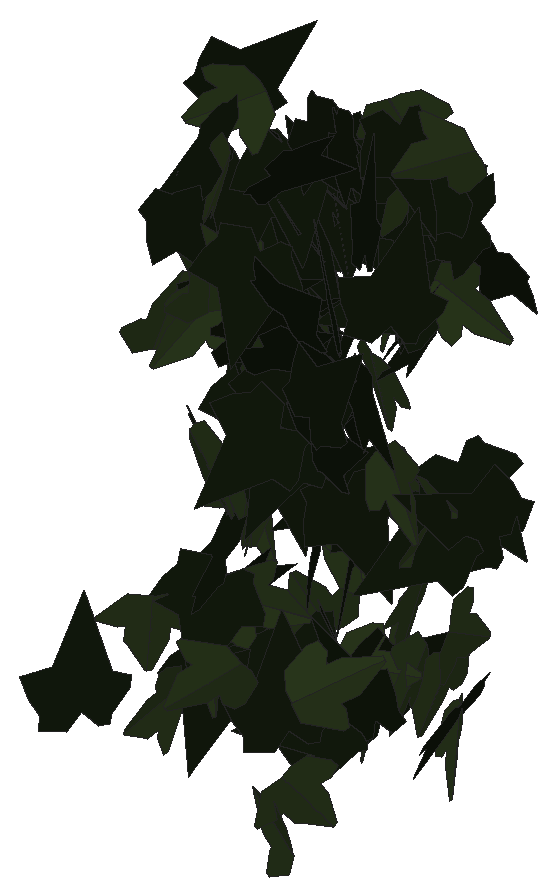
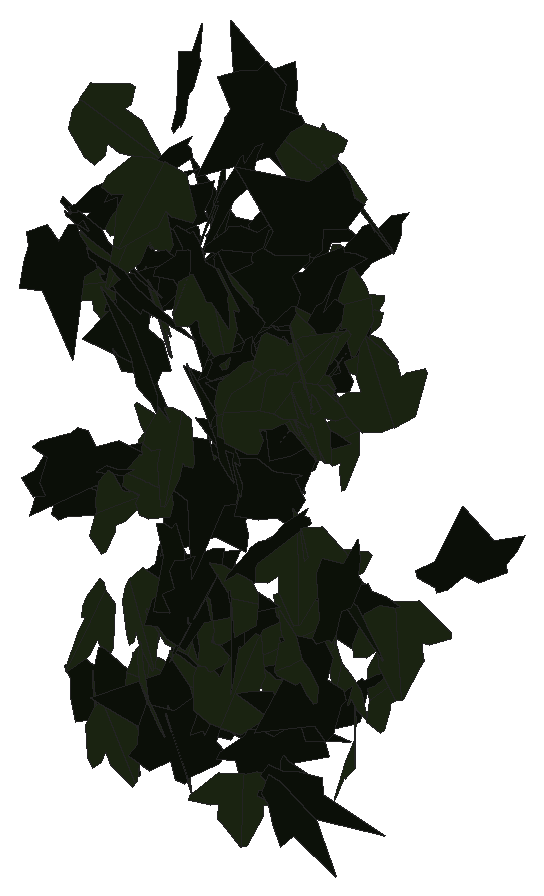
# SketchUp Ruby script. Lengths in inches.
U = 1.inch
M = Sketchup.active_model
def pt(a) = Geom::Point3d.new(a.map { |v| v * U })
def face(e, loops, mat)
  f = e.add_face(loops[0].map { |a| pt(a) })
  loops[1..].each { |l| e.add_face(l.map { |a| pt(a) }).erase! }
  f.material = f.back_material = mat if mat
  f
end
# faces: each face lists its corners as indices into pts; further lists are holes
def faces(e, pts, list, mat = nil) = list.each { |f| face(e, (f[0].is_a?(Array) ? f : [f]).map { |l| l.map { |i| pts[i] } }, mat) }
# xy, xz, yz: faces in a plane at the given z, y or x. An outline is a flat list of corners, or four numbers for a rectangle; further outlines are holes
def ring(l) = l.size == 4 ? [[l[0], l[1]], [l[2], l[1]], [l[2], l[3]], [l[0], l[3]]] : l.each_slice(2).to_a
def flat(e, list, mat, &to3) = list.each { |f| face(e, (f[0].is_a?(Array) ? f : [f]).map { |l| ring(l).map { |u, v| to3.(u, v) } }, mat) }
def xy(e, z, list, mat = nil) = flat(e, list, mat) { |x, y| [x, y, z] }
def xz(e, y, list, mat = nil) = flat(e, list, mat) { |x, z| [x, y, z] }
def yz(e, x, list, mat = nil) = flat(e, list, mat) { |y, z| [x, y, z] }
def lines(e, pts, list) = list.each { |a, b| e.add_line(pt(pts[a]), pt(pts[b])) }
# prism: a flat outline (further loops are holes) pulled along v
def prism(e, loops, v, mat = nil)
  f = face(e, loops, mat); d = Geom::Vector3d.new(v.map { |x| x * U })
  f.pushpull(f.normal.samedirection?(d) ? d.length : -d.length)
end
def box(e, o, s, mat = nil) = prism(e, [[o, [o[0] + s[0], o[1], o[2]], [o[0] + s[0], o[1] + s[1], o[2]], [o[0], o[1] + s[1], o[2]]]], [0, 0, s[2]], mat)
def at(x, y, z, deg = 0) = Geom::Transformation.translation(pt([x, y, z])) * Geom::Transformation.rotation(ORIGIN, Z_AXIS, deg.degrees)
def axes(o, x, y, z) = Geom::Transformation.new([*x, 0, *y, 0, *z, 0, *pt(o).to_a, 1])
def part(name) = M.definitions.add(name)
# library, detail: a bought-in or finely detailed component or shape, given as its bounding box
def library(name, o, s) = part(name).tap { |d| box(d.entities, o, s) }
def detail(e, o, s) = box(e.add_group.entities, o, s)
def put(e, d, t, mat = nil) = e.add_instance(d, t).tap { |i| i.material = mat if mat }
def group(e, t, mat = nil) = e.add_group.tap { |g| g.transformation = t; g.material = mat if mat }.entities
root = M.entities
M.materials.add("efeu1").color = [18, 25, 13]
M.materials.add("efeu2").color = [43, 57, 29]
c1 = part("ivyleaf_9")
p = [[1.54,2.16,1.25],[1.36,2.04,1.19],[-0.21,0.99,0.68],[-0.71,1.11,0.82],[-0.85,0.86,0.67],[-0.8,0.17,0.21],
  [-0.9,-0.01,0.1],[-0.67,-0.16,-0.02],[-0.08,-0.08,-0.05],[-0.03,-0.6,-0.4],[0.65,-0.88,-0.66],[0.83,-0.6,-0.49],
  [1.29,-0.42,-0.43],[1.8125,-0.07,-0.26],[1.21,0.44,0.15]]
faces(c1.entities,p,[[0,1,2,3,4,5,6,7,8,9,10,11,12,13,14]],"efeu1")
c2 = part("ivyleaf_10")
p = [[0,0.5,-0.03],[-0.0625,2.02,-0.43],[-0.19,2.01,-0.46],[-0.54,1.05,-0.29],[-0.52,0.625,-0.18],[-0.83,0.76,-0.28],
  [-1.16,0.64,-0.33],[-1.15,0.33,-0.24],[-0.77,-0.39,0.02],[-0.3,-0.51,0.16],[0.04,-0.48,0.23],[-0.02,2.01,-0.4375],
  [-0.06,2.01,-0.43],[0.04,-0.49,0.23],[0.67,-0.49,0.14],[1.38,0.36,-0.2],[1.375,0.51,-0.24],[0.81,0.65,-0.19],
  [0.62,0.59,-0.15],[0.6,1.09,-0.28],[0.5,1.23,-0.31]]
faces(c2.entities,p,[[0,1,2,3,4,5,6,7,8,9,10],[11,12,0,13,14,15,16,17,18,19,20]],"efeu2")
put(root,c1,axes([35.01,221.78,217.05],[0.13456,-0.26999,0.39875],[0.16922,-0.36111,-0.30161],[0.45084,0.21612,-0.00581]))
put(root,c2,axes([35.25,220.52,219.36],[-0.18393,-0.45885,0.07501],[0.03644,0.06619,0.49426],[-0.46351,0.18729,0.00909]))
put(root,c2,axes([35.36,222.2,220.23],[0.48054,0.03404,-0.13388],[-0.13413,-0.00085,-0.48167],[-0.03302,0.49884,0.00832]))
put(root,c1,axes([35.67,222.1875,214.3125],[-0.42769,-0.02431,0.25786],[-0.25798,-0.00416,-0.42829],[0.02297,-0.49939,-0.00899]))
put(root,c2,axes([35.41,222.34,220.22],[0.05756,0.41296,0.27595],[-0.04863,-0.27177,0.41686],[0.49429,-0.07483,0.00888]))
put(root,c1,axes([35.55,222.26,214.45],[-0.30426,0.30044,-0.25915],[0.17223,-0.1942,-0.42735],[-0.35744,-0.34932,0.01468]))
put(root,c2,axes([35.47,222.05,220.91],[0.25347,-0.43086,0.01047],[0.00775,-0.00759,-0.49988],[0.43092,0.25357,0.00284]))
put(root,c2,axes([35.7,222.04,220.41],[0.21225,0.2584,0.37172],[-0.24741,-0.27761,0.33425],[0.37913,-0.32582,0.01001]))
put(root,c2,axes([35.59,219.91,215.81],[-0.35365,-0.35122,0.03974],[-0.02811,-0.02809,-0.49842],[0.35234,-0.35477,0.00012]))
put(root,c2,axes([35.6875,222.14,220.18],[0.42273,-0.12731,-0.23471],[-0.22624,0.06265,-0.44147],[0.14182,0.47944,-0.00464]))
put(root,c2,axes([35.31,222.22,216.36],[0.27565,-0.05691,0.41325],[0.40121,-0.09944,-0.28132],[0.11421,0.4867,-0.00916]))
put(root,c2,axes([35.55,220.875,214.47],[-0.13494,0.35001,-0.33059],[0.09604,-0.31686,-0.37467],[-0.47177,-0.16462,0.01828]))
put(root,c2,axes([35.78,222.82,220.1],[-0.09609,-0.06927,0.48577],[-0.04461,-0.49171,-0.07894],[0.48865,-0.05852,0.08832]))
put(root,c1,axes([35.47,221.61,222.45],[-0.05533,-0.05972,0.49333],[0.47516,0.13896,0.07012],[-0.14548,0.47657,0.04138]))
put(root,c1,axes([35.78,221.15,215.43],[0.13838,0.29338,0.3805],[0.14932,0.3501,-0.32425],[-0.45668,0.20337,0.00928]))
put(root,c1,axes([35.71,220.23,221.61],[0.15766,-0.33418,-0.33685],[-0.12866,0.31155,-0.3693],[0.45671,0.20313,0.01225]))
put(root,c2,axes([36,220.49,220.04],[0.16571,0.2658,-0.38973],[-0.20211,-0.33324,-0.31321],[-0.42625,0.26134,-0.003]))
put(root,c2,axes([35.93,219.86,214.67],[-0.00988,0.03456,-0.49871],[-0.07298,-0.49356,-0.03275],[-0.49455,0.07215,0.0148]))
put(root,c1,axes([35.77,221.45,219.67],[0.10413,-0.45218,0.18626],[0.03959,-0.18202,-0.46401],[0.48743,0.11138,-0.0021]))
put(root,c1,axes([36.09,217.85,215.47],[-0.32802,-0.23976,0.2914],[0.23696,0.16962,0.4063],[-0.29368,0.40465,0.00235]))
put(root,c1,axes([35.91,221.37,221.5],[-0.11398,-0.48467,-0.04586],[0.01076,0.04458,-0.49789],[0.48672,-0.11449,0.00026]))
put(root,c2,axes([36.29,220.94,222.97],[0.28531,-0.00176,-0.4106],[-0.41049,0.01082,-0.28528],[0.00989,0.49988,0.00473]))
put(root,c2,axes([35.75,220.55,220.79],[-0.25453,0.12719,-0.41114],[0.37694,-0.16461,-0.28428],[-0.20767,-0.45467,-0.01209]))
put(root,c1,axes([36.32,220.41,222.57],[-0.43563,0.24542,-0.00064],[0.00085,0.00021,-0.5],[-0.24542,-0.43563,-0.0006]))
put(root,c1,axes([36.37,220.35,216.59],[-0.34372,0.34921,0.09956],[-0.06978,0.07101,-0.48999],[-0.35635,-0.35073,-0.00008]))
put(root,c2,axes([36.31,222.3125,219.78],[-0.02613,-0.0099,-0.49922],[-0.35119,-0.35499,0.02542],[-0.35494,0.35197,0.0116]))
put(root,c2,axes([36.2,221.17,217.25],[-0.30668,-0.3949,-0.0011],[0.0027,-0.00071,-0.49999],[0.39489,-0.30669,0.00257]))
put(root,c1,axes([36.03,220.64,214.71],[-0.07629,-0.47586,0.13318],[-0.02344,-0.13112,-0.48193],[0.49359,-0.07978,-0.0023]))
put(root,c1,axes([35.74,221.92,221.75],[0.38113,-0.20054,0.25402],[0.22879,-0.11061,-0.4306],[0.2289,0.44447,0.00745]))
put(root,c2,axes([35.93,220.54,215.26],[0.37466,-0.14144,0.29938],[0.28482,-0.09287,-0.40032],[0.16885,0.4705,0.01098]))
put(root,c2,axes([36.16,220.38,220.25],[-0.20375,-0.45,-0.07737],[-0.02016,-0.07578,0.49381],[-0.45616,0.20435,0.01274]))
put(root,c1,axes([35.9,220.68,219.92],[0.16039,0.03716,0.47212],[0.4564,0.1209,-0.16457],[-0.12639,0.48374,0.00487]))
put(root,c1,axes([35.82,221.51,219.67],[0.21229,0.13832,-0.43105],[0.36086,0.23576,0.25337],[0.27333,-0.41867,0.00027]))
put(root,c1,axes([36.23,222.23,220.61],[-0.22899,-0.4393,0.06766],[-0.02428,-0.06364,-0.49534],[0.44382,-0.23014,0.00781]))
put(root,c1,axes([36.57,222.07,221.07],[-0.05323,0.10318,0.48633],[-0.24972,0.41739,-0.11589],[-0.42989,-0.25523,0.0071]))
put(root,c1,axes([36.23,220.45,216.17],[-0.29292,-0.3919,-0.10304],[0.07113,0.07544,-0.48913],[0.39892,-0.30121,0.01156]))
put(root,c1,axes([36.2,221.38,220.15],[-0.1026,-0.40095,-0.28055],[0.09172,0.26582,-0.41344],[0.48069,-0.1363,0.01901]))
put(root,c1,axes([36.1875,221.75,217.62],[0.09283,-0.47949,-0.10711],[-0.01877,0.10546,-0.48839],[0.49095,0.09469,0.00158]))
put(root,c1,axes([36.77,221.64,214.77],[-0.36053,-0.00774,0.34635],[-0.34545,-0.02968,-0.36025],[0.02613,-0.49906,0.01606]))
put(root,c2,axes([36.49,220.81,217.3],[0.28484,-0.36067,-0.19693],[-0.08843,0.1802,-0.45794],[0.40131,0.29571,0.03887]))
put(root,c1,axes([36.22,221.68,221.23],[0.43983,-0.2275,-0.06921],[-0.0612,0.03234,-0.49519],[0.22979,0.44407,0.0006]))
put(root,c2,axes([36.37,222.05,214.07],[0.36359,0.34266,0.01964],[0.01349,0.01432,-0.49961],[-0.34296,0.36384,0.00117]))
put(root,c1,axes([36.33,221.49,214.53],[-0.10411,-0.41087,-0.26523],[0.07854,0.25361,-0.42369],[0.48269,-0.12989,0.01174]))
put(root,c2,axes([36.3,220.73,215.8125],[0.11924,0.12869,0.46821],[0.19159,0.43053,-0.16713],[-0.44618,0.21927,0.05336]))
put(root,c2,axes([36.6,220.03,222.5],[0.29929,-0.38018,-0.12605],[-0.07724,0.09962,-0.48385],[0.39301,0.3091,0.0009]))
put(root,c1,axes([36.51,221.1,218.76],[-0.26653,-0.40408,-0.12522],[0.0652,0.10699,-0.48405],[0.41798,-0.27436,-0.00434]))
put(root,c2,axes([36.33,219.99,218.38],[-0.25445,0.2018,-0.38017],[0.29197,-0.24356,-0.3247],[-0.31624,-0.38724,0.00611]))
put(root,c2,axes([36.81,222.24,221.3],[-0.44574,-0.07255,0.2146],[-0.2119,-0.0339,-0.45161],[0.08008,-0.49355,-0.00052]))
put(root,c2,axes([36.7,221.99,215.09],[-0.27068,-0.3366,-0.25186],[-0.15994,-0.19458,0.43193],[-0.38878,0.31439,-0.00233]))
put(root,c1,axes([36.31,221.84,220.84],[-0.10538,-0.14066,-0.46809],[0.42654,0.20735,-0.15833],[0.23866,-0.43269,0.07629]))
put(root,c1,axes([36.49,221.61,221.96],[-0.17253,-0.4128,-0.22323],[0.10957,0.19583,-0.44682],[0.45632,-0.2031,0.02289]))
put(root,c1,axes([36.91,221.51,216.48],[0.00786,0.0042,-0.49992],[-0.45572,0.20565,-0.00544],[0.20557,0.45573,0.00706]))
put(root,c1,axes([36.48,220.41,219.81],[0.12495,0.38033,-0.29956],[0.06196,0.29427,0.39946],[0.48015,-0.13695,0.02641]))
put(root,c1,axes([36.5,222.03,219.83],[0.10211,-0.35561,0.33632],[0.09972,-0.32124,-0.36995],[0.4792,0.14263,0.00531]))
put(root,c2,axes([36.81,221.11,219.64],[-0.24635,-0.40321,-0.16352],[0.08919,0.13712,-0.47249],[0.42586,-0.26196,0.00436]))
put(root,c1,axes([36.97,222.63,217.01],[-0.08948,-0.05815,-0.48848],[0.02143,-0.49648,0.05518],[-0.49146,-0.01107,0.09135]))
put(root,c2,axes([36.5,222.03,216.75],[0.03504,-0.03536,-0.49752],[0.49358,0.07425,0.02949],[0.0718,-0.49319,0.0401]))
put(root,c2,axes([37.19,219.41,215.69],[-0.22668,-0.21496,0.3904],[-0.29784,-0.25275,-0.31211],[0.33152,-0.37405,-0.01346]))
put(root,c1,axes([36.68,222.48,221.85],[-0.18677,-0.07923,-0.45699],[0.45455,0.06668,-0.19733],[0.09222,-0.48916,0.04712]))
put(root,c1,axes([36.99,221.93,218.52],[0.37446,0.05429,-0.32685],[-0.32677,-0.02106,-0.37786],[-0.0548,0.4966,0.01971]))
put(root,c1,axes([36.7,220.68,217.92],[0.20781,0.43016,-0.14758],[0.06421,0.13288,0.47773],[0.45021,-0.2175,-0.00001]))
put(root,c1,axes([36.87,221.67,218.56],[-0.13441,0.41242,0.24869],[0.05879,-0.24221,0.43345],[0.47799,0.14576,0.01661]))
put(root,c1,axes([36.92,222.125,221.63],[-0.24113,-0.36609,-0.2405],[0.13124,0.20154,-0.43836],[0.41789,-0.27453,-0.0011]))
put(root,c1,axes([36.81,222.54,216.61],[0.24478,-0.19865,-0.3881],[0.2956,-0.25154,0.31519],[-0.32047,-0.38375,-0.0057]))
put(root,c1,axes([36.98,221.34,222.63],[0.23541,-0.24923,-0.36396],[-0.2544,0.26032,-0.3428],[0.36037,0.34658,-0.00424]))
put(root,c1,axes([37.03,221.85,222.25],[0.29545,-0.18178,-0.36009],[-0.30181,0.19651,-0.34683],[0.26762,0.4223,0.0064]))
put(root,c2,axes([37.17,222.16,215.91],[0.46311,0.08908,0.16611],[-0.16527,-0.02,0.47147],[0.09065,-0.49159,0.01092]))
put(root,c1,axes([37.11,220.13,221.33],[-0.35485,-0.31194,-0.16362],[0.12272,0.10821,-0.47247],[0.33018,-0.37548,-0.00024]))
put(root,c1,axes([37.22,220.74,218.51],[-0.45309,-0.16224,-0.13561],[0.12757,0.046,-0.48126],[0.16864,-0.4707,-0.00028]))
put(root,c1,axes([37.25,220.32,218.78],[-0.31351,-0.33549,0.19788],[-0.12223,-0.15645,-0.45889],[0.36983,-0.33611,0.01608]))
put(root,c1,axes([37.02,220.65,219.37],[-0.01592,-0.2587,-0.42758],[0.07691,0.42143,-0.25784],[0.49379,-0.07398,0.02637]))
put(root,c1,axes([37.69,221.2,214.375],[-0.35458,-0.04549,0.34958],[-0.34279,-0.07123,-0.35696],[0.08228,-0.4928,0.01933]))
put(root,c1,axes([37.03,221.84,221.07],[0.10036,-0.07068,-0.4847],[0.47276,-0.11546,0.11473],[-0.12815,-0.48132,0.04366]))
put(root,c1,axes([37.48,221.94,216.79],[-0.00253,0.21702,0.45044],[0.01399,0.4503,-0.21687],[-0.4998,0.01151,-0.00835]))
put(root,c1,axes([37.22,222.03,216.67],[-0.17213,0.07658,-0.46315],[0.414,-0.20779,-0.18822],[-0.22131,-0.44828,0.00813]))
put(root,c1,axes([37.08,220.72,218.34],[-0.11282,-0.00573,0.48707],[0.48582,-0.03758,0.11209],[0.03532,0.49855,0.01405]))
put(root,c2,axes([37.44,222.14,218.97],[-0.4564,0.19198,0.06956],[-0.06539,0.02393,-0.49513],[-0.19344,-0.46105,0.00327]))
put(root,c1,axes([37.09,221.79,214.97],[0.12826,-0.25659,0.40952],[0.16489,-0.37504,-0.28663],[0.45427,0.20858,-0.01159]))
put(root,c1,axes([37.53,220.21,214.67],[-0.44788,-0.12982,0.18042],[0.18076,0.02343,0.46559],[-0.12934,0.48228,0.02594]))
put(root,c1,axes([37.25,220.15,220.05],[0.39119,0.27523,0.14566],[0.11446,0.09043,-0.47825],[-0.2896,0.40752,0.00775]))
put(root,c1,axes([37.56,222.02,214.08],[0.13039,0.09481,0.4733],[-0.40991,-0.23714,0.16043],[0.25489,-0.42986,0.01589]))
put(root,c2,axes([37.55,222,214.46],[0.30567,-0.37979,0.11102],[0.07392,-0.083,-0.48749],[0.38872,0.31443,0.00541]))
put(root,c1,axes([37.51,219.96,222.71],[0.25003,0.33159,0.27844],[0.15182,0.23398,-0.41498],[-0.4055,0.29206,0.01632]))
put(root,c2,axes([37.65,222.3,222.66],[-0.39526,-0.23135,-0.20062],[0.17627,0.09597,-0.45795],[0.2504,-0.43274,0.0057]))
put(root,c2,axes([37.55,222.59,215.34],[0.30843,-0.21713,0.32821],[0.25524,-0.20703,-0.37682],[0.29954,0.39999,-0.01686]))
put(root,c1,axes([37.58,221.67,214.64],[0.09308,0.07847,0.48495],[0.39227,0.28526,-0.12145],[-0.29573,0.40308,-0.00846]))
put(root,c1,axes([37.6,221.3,217.53],[-0.16981,-0.20881,-0.42138],[0.31331,0.28388,-0.26693],[0.35072,-0.3547,0.03443]))
put(root,c2,axes([37.49,221.65,214.9],[0.06926,-0.08453,-0.48791],[0.48165,-0.10287,0.0862],[-0.11496,-0.48195,0.06718]))
put(root,c1,axes([38.36,222.31,220.99],[-0.37146,0.1981,0.26977],[-0.24909,0.10556,-0.42049],[-0.22355,-0.44678,0.02027]))
put(root,c1,axes([37.91,222.13,219.71],[-0.1768,0.43791,0.16425],[0.01378,-0.17064,0.46978],[0.46749,0.17064,0.04827]))
put(root,c2,axes([38.36,219.05,213.79],[-0.0713,0.05399,-0.49194],[-0.35659,0.33903,0.08889],[0.34316,0.36351,-0.00984]))
put(root,c2,axes([38.14,222.59,214.6875],[-0.0622,-0.47456,0.14464],[-0.00553,-0.1451,-0.47845],[0.49608,-0.06112,0.0128]))
put(root,c1,axes([37.97,221.87,221.27],[-0.32515,-0.10967,-0.36367],[0.34397,0.11808,-0.34314],[0.16114,-0.47332,-0.00134]))
put(root,c2,axes([38.09,221.75,220.64],[0.34729,-0.3558,0.05283],[0.03639,-0.0383,-0.4972],[0.35786,0.34919,-0.00071]))
put(root,c1,axes([37.77,220.44,218.71],[0.06331,-0.07543,0.49021],[0.32311,-0.36865,-0.09845],[0.37628,0.32925,0.00207]))
put(root,c1,axes([37.94,221.97,222.63],[0.10056,-0.45864,-0.17187],[-0.01842,0.17179,-0.4692],[0.48944,0.1007,0.01765]))
put(root,c2,axes([38.11,221.99,221.85],[-0.10019,-0.38845,-0.29844],[0.11377,0.27783,-0.39983],[0.47646,-0.14802,0.03272]))
put(root,c1,axes([38.43,221.85,220.49],[-0.33172,-0.14869,0.3433],[-0.29739,-0.17357,-0.36254],[0.22698,-0.44471,0.02672]))
put(root,c1,axes([38.24,221.74,220],[-0.21384,0.36613,-0.265],[-0.13294,0.22924,0.424],[0.43197,0.25179,-0.00069]))
put(root,c1,axes([38.4375,222,220.02],[-0.36926,0.33285,-0.05347],[0.03999,-0.03549,-0.49713],[-0.33474,-0.37142,-0.00041]))
put(root,c2,axes([38.25,221.9,216.12],[0.11579,-0.48512,0.03543],[0.00676,-0.03481,-0.49874],[0.48636,0.11598,-0.00151]))
put(root,c1,axes([38.41,220.08,220.68],[0.02985,-0.23167,0.44208],[-0.0791,0.43508,0.23334],[-0.4928,-0.08387,-0.01068]))
put(root,c2,axes([38.17,221.99,215.03],[0.05261,-0.26268,0.42218],[0.21518,-0.37069,-0.25746],[0.44825,0.20878,0.07404]))
put(root,c1,axes([38.6,222.31,221.88],[-0.19495,-0.41079,-0.20796],[-0.09415,-0.1855,0.45467],[-0.4507,0.21643,-0.00503]))
put(root,c2,axes([38.39,219.21,214.56],[-0.21739,-0.34159,-0.29335],[0.1739,0.23678,-0.40459],[0.41533,-0.27794,0.01586]))
put(root,c2,axes([38.11,221.63,217.71],[-0.01185,-0.03736,0.49846],[0.49204,0.08695,0.01822],[-0.08805,0.49096,0.0347]))
put(root,c2,axes([38.23,221.35,218.13],[0.35751,-0.05917,0.34451],[0.3461,-0.00915,-0.36074],[0.04899,0.4964,0.03441]))
put(root,c1,axes([38.8125,220.31,215.22],[0.11917,-0.11323,0.4722],[-0.35951,0.30627,0.16417],[-0.32642,-0.37865,-0.00841]))
put(root,c1,axes([38.97,222.2,221.5625],[-0.43944,0.1812,0.15512],[-0.14439,0.05675,-0.47532],[-0.18986,-0.46254,0.00245]))
put(root,c2,axes([38.75,221.93,217.29],[0.01137,0.11449,-0.48658],[-0.10023,-0.4763,-0.11442],[-0.48972,0.10014,0.01212]))
put(root,c2,axes([39.14,221.65,222.84],[-0.1938,-0.11519,0.44629],[-0.38489,-0.2259,-0.22545],[0.25357,-0.43093,-0.00112]))
put(root,c1,axes([39.04,221.61,217.35],[-0.41639,-0.19828,0.19314],[-0.16844,-0.09535,-0.46102],[0.21965,-0.44899,0.01261]))
put(root,c1,axes([39,221.8,214.73],[-0.23174,0.41125,-0.16482],[0.07959,-0.14433,-0.47205],[-0.43584,-0.24503,0.00143]))
put(root,c1,axes([38.6,219.35,219.91],[-0.15787,0.17518,0.4409],[0.29057,-0.33162,0.2358],[0.37503,0.33067,0.0029]))
put(root,c2,axes([38.87,221.88,215.77],[0.02944,-0.26213,-0.42476],[0.03782,0.42545,-0.25993],[0.4977,-0.01682,0.04488]))
put(root,c1,axes([38.9,220.57,220.83],[-0.30664,-0.16528,0.35868],[0.31674,0.16832,0.34834],[-0.23589,0.44085,0.00147]))
put(root,c2,axes([38.7,222.09,214.35],[0.31578,-0.2128,0.32403],[0.26542,-0.18593,-0.38077],[0.28255,0.41249,-0.00446]))
put(root,c1,axes([38.65,218.75,221.64],[-0.08314,-0.11251,0.48003],[0.33379,-0.37112,-0.02918],[0.36287,0.31561,0.13682]))
put(root,c1,axes([39.13,219.76,222.3125],[-0.02148,-0.18733,0.46309],[0.07187,0.45753,0.18841],[-0.49434,0.07465,0.00727]))
put(root,c1,axes([39.21,222.31,221.14],[0.25525,0.13461,-0.40832],[-0.39666,-0.10945,-0.28404],[-0.16585,0.46894,0.05092]))
put(root,c1,axes([38.91,221.97,218.11],[-0.05015,-0.26372,-0.42183],[0.15522,0.39451,-0.26509],[0.47264,-0.15754,0.04229]))
put(root,c2,axes([38.77,221.89,220.6],[0.16762,0.03454,0.4698],[0.44668,0.14671,-0.17016],[-0.14961,0.47674,0.01832]))
put(root,c1,axes([39.42,222.01,217.3],[-0.05639,0.00649,0.49677],[-0.46383,-0.1798,-0.0503],[0.17799,-0.46651,0.0263]))
put(root,c1,axes([38.85,219.97,220.12],[0.07338,-0.0728,-0.4892],[0.49456,0.00572,0.07333],[-0.00508,-0.49464,0.07285]))
put(root,c2,axes([39.02,218.79,216.3],[0.15631,0.09036,-0.46626],[0.38694,0.26041,0.18018],[0.2754,-0.41716,0.01149]))
